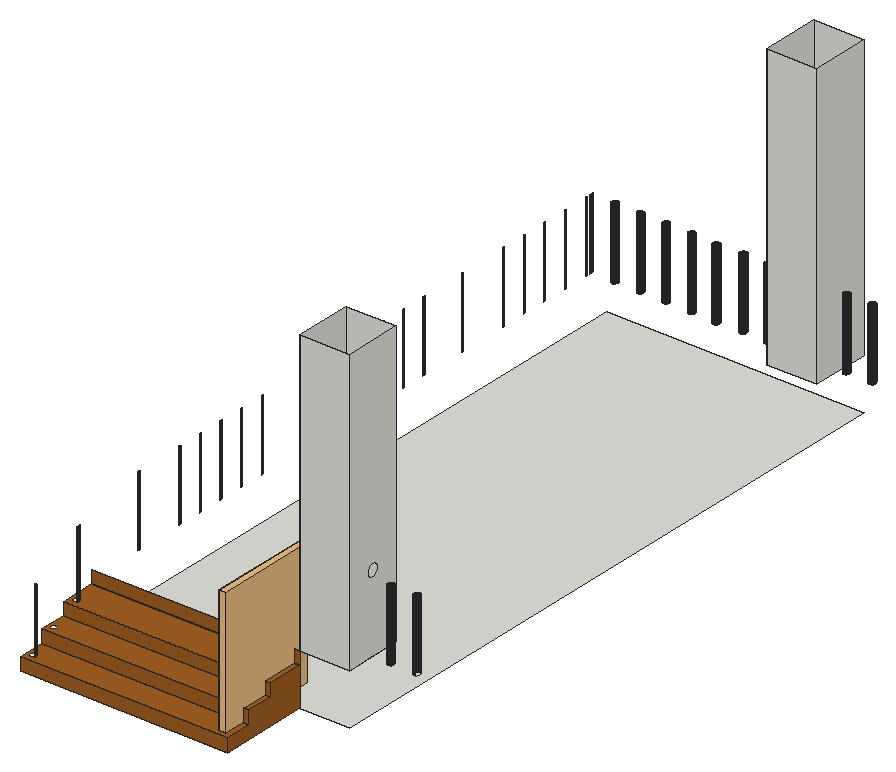
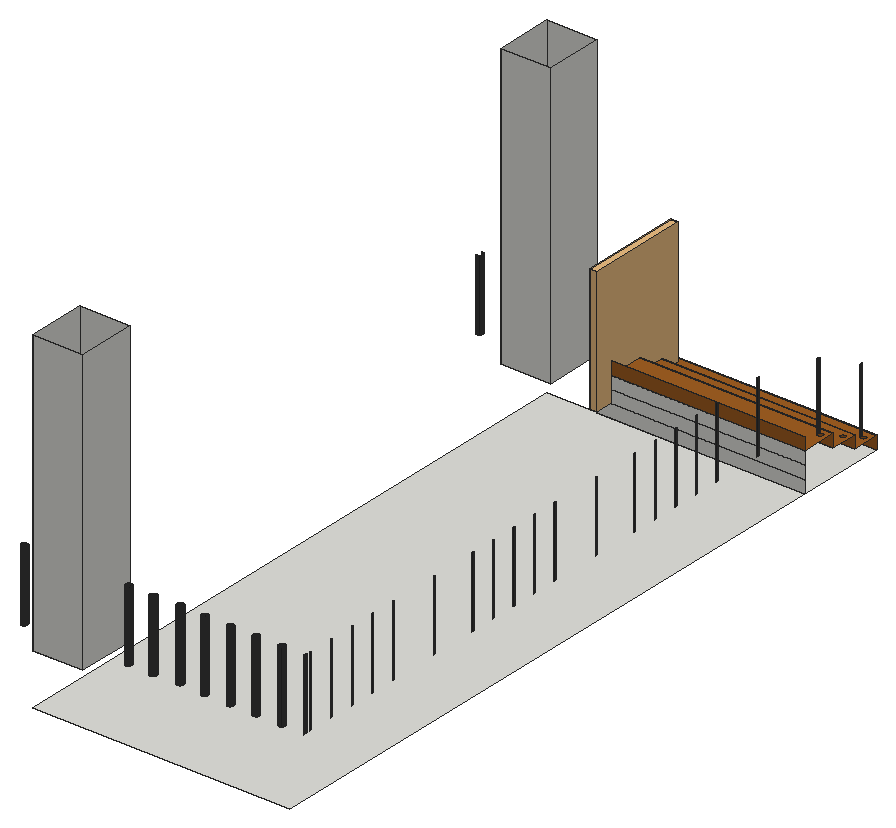
# SketchUp Ruby script. Lengths in inches.
U = 1.inch
M = Sketchup.active_model
def pt(a) = Geom::Point3d.new(a.map { |v| v * U })
def face(e, loops, mat)
  f = e.add_face(loops[0].map { |a| pt(a) })
  loops[1..].each { |l| e.add_face(l.map { |a| pt(a) }).erase! }
  f.material = f.back_material = mat if mat
  f
end
# faces: each face lists its corners as indices into pts; further lists are holes
def faces(e, pts, list, mat = nil) = list.each { |f| face(e, (f[0].is_a?(Array) ? f : [f]).map { |l| l.map { |i| pts[i] } }, mat) }
# xy, xz, yz: faces in a plane at the given z, y or x. An outline is a flat list of corners, or four numbers for a rectangle; further outlines are holes
def ring(l) = l.size == 4 ? [[l[0], l[1]], [l[2], l[1]], [l[2], l[3]], [l[0], l[3]]] : l.each_slice(2).to_a
def flat(e, list, mat, &to3) = list.each { |f| face(e, (f[0].is_a?(Array) ? f : [f]).map { |l| ring(l).map { |u, v| to3.(u, v) } }, mat) }
def xy(e, z, list, mat = nil) = flat(e, list, mat) { |x, y| [x, y, z] }
def xz(e, y, list, mat = nil) = flat(e, list, mat) { |x, z| [x, y, z] }
def yz(e, x, list, mat = nil) = flat(e, list, mat) { |y, z| [x, y, z] }
def lines(e, pts, list) = list.each { |a, b| e.add_line(pt(pts[a]), pt(pts[b])) }
# prism: a flat outline (further loops are holes) pulled along v
def prism(e, loops, v, mat = nil)
  f = face(e, loops, mat); d = Geom::Vector3d.new(v.map { |x| x * U })
  f.pushpull(f.normal.samedirection?(d) ? d.length : -d.length)
end
def box(e, o, s, mat = nil) = prism(e, [[o, [o[0] + s[0], o[1], o[2]], [o[0] + s[0], o[1] + s[1], o[2]], [o[0], o[1] + s[1], o[2]]]], [0, 0, s[2]], mat)
def at(x, y, z, deg = 0) = Geom::Transformation.translation(pt([x, y, z])) * Geom::Transformation.rotation(ORIGIN, Z_AXIS, deg.degrees)
def axes(o, x, y, z) = Geom::Transformation.new([*x, 0, *y, 0, *z, 0, *pt(o).to_a, 1])
def part(name) = M.definitions.add(name)
# library, detail: a bought-in or finely detailed component or shape, given as its bounding box
def library(name, o, s) = part(name).tap { |d| box(d.entities, o, s) }
def detail(e, o, s) = box(e.add_group.entities, o, s)
def put(e, d, t, mat = nil) = e.add_instance(d, t).tap { |i| i.material = mat if mat }
def group(e, t, mat = nil) = e.add_group.tap { |g| g.transformation = t; g.material = mat if mat }.entities
root = M.entities
M.materials.add("[0137_Black]").color = [45, 45, 45]
M.materials.add("[Wood Square Tile 02]").color = [160, 95, 34]
xy(root,0,[[0,0,193.3125,84],[0,84,240,684]])
xy(root,12,[[[0,0,193.3125,25.4375],[5.2,5.16,4.89,5.1875,4.58,5.25,4.28,5.34,3.99,5.47,3.72,5.62,3.46,5.8,3.23,6.01,3.01,6.24,2.83,6.49,2.67,6.76,2.53,7.05,2.43,7.35,2.37,7.65,2.33,7.96,2.33,8.28,2.36,8.59,2.42,8.9,2.51,9.2,2.64,9.49,2.79,9.76,2.97,10.02,3.18,10.25,3.41,10.47,3.66,10.65,3.93,10.8125,4.22,10.94,4.52,11.04,4.82,11.11,5.13,11.15,5.45,11.15,5.76,11.12,6.07,11.0625,6.37,10.97,6.66,10.84,6.93,10.6875,7.1875,10.51,7.42,10.3,7.63,10.07,7.82,9.82,7.98,9.55,8.11,9.26,8.21,8.96,8.28,8.66,8.32,8.34,8.32,8.03,8.29,7.72,8.23,7.41,8.14,7.11,8.01,6.82,7.86,6.55,7.68,6.29,7.47,6.06,7.24,5.84,6.99,5.66,6.71,5.5,6.43,5.37,6.13,5.27,5.83,5.2,5.51,5.16]]],"[Wood Square Tile 02]")
xy(root,24,[[[0,25.4375,193.3125,50.75],[4.7,30.03,4.39,30.06,4.08,30.12,3.78,30.22,3.49,30.34,3.22,30.49,2.96,30.68,2.73,30.88,2.51,31.11,2.33,31.37,2.17,31.64,2.04,31.92,1.9375,32.22,1.87,32.53,1.83,32.84,1.83,33.15,1.86,33.46,1.92,33.77,2.01,34.07,2.14,34.36,2.29,34.63,2.47,34.89,2.68,35.125,2.91,35.34,3.16,35.53,3.43,35.6875,3.72,35.82,4.02,35.92,4.32,35.99,4.63,36.02,4.95,36.03,5.26,36,5.57,35.93,5.87,35.84,6.16,35.72,6.43,35.5625,6.6875,35.38,6.92,35.17,7.14,34.94,7.32,34.6875,7.48,34.42,7.61,34.13,7.71,33.84,7.78,33.53,7.82,33.22,7.82,32.9,7.79,32.59,7.73,32.28,7.64,31.98,7.51,31.7,7.36,31.42,7.18,31.17,6.97,30.93,6.74,30.72,6.49,30.53,6.22,30.37,5.93,30.24,5.63,30.14,5.33,30.07,5.01,30.03]]],"[Wood Square Tile 02]")
xy(root,36,[[[0,50.75,193.3125,84],[5.56,55.09,5.25,55.12,4.94,55.18,4.64,55.27,4.35,55.4,4.08,55.55,3.82,55.74,3.59,55.94,3.375,56.17,3.1875,56.43,3.03,56.7,2.9,56.98,2.8,57.28,2.73,57.59,2.69,57.9,2.6875,58.21,2.72,58.52,2.78,58.83,2.87,59.13,3,59.42,3.15,59.69,3.33,59.95,3.54,60.19,3.77,60.4,4.02,60.59,4.29,60.75,4.58,60.875,4.875,60.98,5.18,61.05,5.49,61.08,5.81,61.08,6.12,61.06,6.43,60.99,6.73,60.9,7.02,60.78,7.29,60.62,7.55,60.4375,7.78,60.23,7.99,60,8.18,59.75,8.34,59.48,8.47,59.19,8.57,58.9,8.64,58.59,8.68,58.28,8.68,57.96,8.65,57.65,8.59,57.34,8.5,57.04,8.37,56.75,8.22,56.48,8.04,56.23,7.83,55.99,7.6,55.78,7.35,55.59,7.08,55.43,6.79,55.3,6.49,55.2,6.1875,55.13,5.875,55.09]]],"[Wood Square Tile 02]")
xy(root,48,[[193.3125,84,240,138.5625],[257.12,108.28,257.9,108.38,258.62,108.68,259.24,109.16,259.72,109.78,260.02,110.5,260.12,111.28,260.02,112.06,259.72,112.78,259.24,113.4,258.62,113.88,257.9,114.18,257.12,114.28,256.34,114.18,255.62,113.88,255,113.4,254.52,112.78,254.22,112.06,254.12,111.28,254.22,110.5,254.52,109.78,255,109.16,255.62,108.68,256.34,108.38],[281.12,108.28,280.34,108.38,279.62,108.68,279,109.16,278.52,109.78,278.22,110.5,278.12,111.28,278.22,112.06,278.52,112.78,279,113.4,279.62,113.88,280.34,114.18,281.12,114.28,281.9,114.18,282.62,113.88,283.24,113.4,283.72,112.78,284.02,112.06,284.12,111.28,284.02,110.5,283.72,109.78,283.24,109.16,282.62,108.68,281.9,108.38],[193.3125,629.4375,240,684],[246.01,653.72,246.79,653.82,247.51,654.12,248.13,654.6,248.61,655.22,248.91,655.94,249.01,656.72,243.01,656.72,243.11,655.94,243.41,655.22,243.89,654.6,244.51,654.12,245.23,653.82],
  [270.01,653.72,270.79,653.82,271.51,654.12,272.13,654.6,272.61,655.22,272.91,655.94,273.01,656.72,267.01,656.72,267.11,655.94,267.41,655.22,267.89,654.6,268.51,654.12,269.23,653.82],[243.01,656.72,249.01,656.72,248.91,657.5,248.61,658.22,248.13,658.84,247.51,659.32,246.79,659.62,246.01,659.72,245.23,659.62,244.51,659.32,243.89,658.84,243.41,658.22,243.11,657.5],[267.01,656.72,273.01,656.72,272.91,657.5,272.61,658.22,272.13,658.84,271.51,659.32,270.79,659.62,270.01,659.72,269.23,659.62,268.51,659.32,267.89,658.84,267.41,658.22,267.11,657.5]])
xz(root,0,[[0,0,193.3125,12]],"[Wood Square Tile 02]")
xz(root,25.4375,[[0,12,193.3125,24]],"[Wood Square Tile 02]")
xz(root,50.75,[[0,24,193.3125,36]],"[Wood Square Tile 02]")
xz(root,84,[[0,0,193.3125,12],[0,12,193.3125,24],[0,24,193.3125,36],[193.3125,48,240,312]])
xz(root,84,[[0,36,193.3125,48]],"[Wood Square Tile 02]")
xz(root,138.5625,[[193.3125,48,240,312]])
xz(root,629.4375,[[193.3125,48,240,312]])
xz(root,684,[[193.3125,48,240,312]])
yz(root,8.32,[[8.03,12,8.34,12,8.34,71.9,8.03,72.08]],"[0137_Black]")
yz(root,8.68,[[57.96,36,58.28,98.83]],"[0137_Black]")
yz(root,193.3125,[[84,48,138.5625,312],[629.4375,48,684,312]])
yz(root,193.3125,[[0,0,84,0,84,36,50.75,36,50.75,24,25.4375,24,25.4375,12,0,12]],"[Wood Square Tile 02]")
yz(root,240,[[84,48,111.28,48,111.28,114,110.65,114.03,110.03,114.13,109.43,114.29,108.84,114.52,108.28,114.8,107.75,115.15,107.27,115.54,106.82,115.99,106.43,116.47,106.09,117,105.8,117.56,105.57,118.15,105.41,118.75,105.3125,119.37,105.28,120,105.3125,120.63,105.41,121.25,105.57,121.85,105.8,122.44,106.09,123,106.43,123.53,106.82,124.01,107.27,124.46,107.75,124.85,108.28,125.2,108.84,125.48,109.43,125.71,110.03,125.87,110.65,125.97,111.28,126,111.91,125.97,112.53,125.87,113.14,125.71,113.72,125.48,114.28,125.2,114.81,124.85,115.3,124.46,115.74,124.01,116.14,123.53,116.48,123,116.76,122.44,116.99,121.85,117.15,121.25,117.25,120.63,117.28,120,117.25,119.37,117.15,118.75,116.99,118.15,116.76,117.56,116.48,117,116.14,116.47,115.74,115.99,115.3,115.54,114.81,115.15,114.28,114.8,113.72,114.52,113.14,114.29,112.53,114.13,111.91,114.03,111.28,114,111.28,48,138.5625,48,138.5625,312,84,312],[629.4375,48,684,312]])
p = [[8.01,6.82,12],[8.14,7.11,12],[8.14,7.11,72.59],[8.01,6.82,72.76],[8.23,7.41,12],[8.23,7.41,72.43],
  [8.29,7.72,12],[8.29,7.72,72.25],[8.32,8.03,12],[8.32,8.03,72.08],[8.32,8.34,12],[8.28,8.66,12],
  [8.28,8.66,71.72],[8.32,8.34,71.9],[8.21,8.96,12],[8.21,8.96,71.55],[8.11,9.26,12],[8.11,9.26,71.38],
  [7.98,9.55,12],[7.98,9.55,71.22],[8.04,56.23,36],[8.22,56.48,36],[8.22,56.48,98.83],[8.04,56.23,98.83],
  [8.37,56.75,36],[8.37,56.75,98.83],[8.5,57.04,36],[8.5,57.04,98.83],[8.59,57.34,36],[8.59,57.34,98.83],
  [8.65,57.65,36],[8.65,57.65,98.83],[8.68,57.96,36],[8.68,57.96,98.83],[8.68,58.28,36],[8.64,58.59,36],
  [8.64,58.59,98.83],[8.68,58.28,98.83],[8.57,58.9,36],[8.57,58.9,98.83],[8.47,59.19,36],[8.47,59.19,98.83],
  [8.34,59.48,36],[8.34,59.48,98.83],[8.18,59.75,36],[8.18,59.75,98.83],[7.99,60,36],[7.99,60,98.83],
  [256.34,108.38,48],[257.12,108.28,48],[257.12,108.28,113.8],[256.34,108.38,113.8],[257.9,108.38,48],[257.9,108.38,113.8],
  [280.34,108.38,48],[281.12,108.28,48],[281.12,108.28,113.8],[280.34,108.38,113.8],[281.9,108.38,48],[281.9,108.38,113.8],
  [255.62,108.68,48],[255.62,108.68,113.8],[258.62,108.68,48],[258.62,108.68,113.8],[279.62,108.68,48],[279.62,108.68,113.8],
  [255,109.16,48],[255,109.16,113.8],[259.24,109.16,48],[259.24,109.16,113.8],[279,109.16,48],[279,109.16,113.8],
  [254.52,109.78,48],[254.52,109.78,113.8],[259.72,109.78,48],[259.72,109.78,113.8],[278.52,109.78,48],[278.52,109.78,113.8],
  [254.22,110.5,48],[254.22,110.5,113.8],[260.02,110.5,48],[260.02,110.5,113.8],[278.22,110.5,48],[278.22,110.5,113.8],
  [254.12,111.28,48],[254.12,111.28,113.8],[260.12,111.28,48],[260.12,111.28,113.8],[278.12,111.28,48],[278.12,111.28,113.8],
  [254.22,112.06,48],[254.22,112.06,113.8],[260.02,112.06,48],[260.02,112.06,113.8],[278.22,112.06,48],[278.22,112.06,113.8],
  [254.52,112.78,48],[254.52,112.78,113.8],[259.72,112.78,48],[259.72,112.78,113.8],[278.52,112.78,48],[278.52,112.78,113.8],
  [255,113.4,48],[255,113.4,113.8],[259.24,113.4,48],[259.24,113.4,113.8],[279,113.4,48],[279,113.4,113.8],
  [255.62,113.88,48],[255.62,113.88,113.8],[258.62,113.88,48],[258.62,113.88,113.8],[279.62,113.88,48],[279.62,113.88,113.8],
  [256.34,114.18,48],[256.34,114.18,113.8],[257.9,114.18,48],[257.9,114.18,113.8],[280.34,114.18,48],[280.34,114.18,113.8],
  [282.62,113.88,48],[281.9,114.18,48],[281.9,114.18,113.8],[282.62,113.88,113.8],[257.12,114.28,48],[257.12,114.28,113.8],
  [281.12,114.28,48],[281.12,114.28,113.8],[7.9,127.49,48],[8,128.27,48],[8,128.27,113.8],[7.9,127.49,113.8],
  [7.9,129.05,48],[7.9,129.05,113.8],[7.9,175.49,48],[8,176.27,48],[8,176.27,113.8],[7.9,175.49,113.8],
  [7.9,177.05,48],[7.9,177.05,113.8],[7.9,199.49,48],[8,200.27,48],[8,200.27,113.8],[7.9,199.49,113.8],
  [7.9,201.05,48],[7.9,201.05,113.8],[7.9,223.49,48],[8,224.27,48],[8,224.27,113.8],[7.9,223.49,113.8],
  [7.9,225.05,48],[7.9,225.05,113.8],[7.9,247.49,48],[8,248.27,48],[8,248.27,113.8],[7.9,247.49,113.8],
  [7.9,249.05,48],[7.9,249.05,113.8],[7.9,271.49,48],[8,272.27,48],[8,272.27,113.8],[7.9,271.49,113.8],
  [7.9,273.05,48],[7.9,273.05,113.8],[7.9,316.38,48],[8,317.16,48],[8,317.16,113.8],[7.9,316.38,113.8],
  [7.9,317.93,48],[7.9,317.93,113.8],[7.9,364.38,48],[8,365.16,48],[8,365.16,113.8],[7.9,364.38,113.8],
  [7.9,365.93,48],[7.9,365.93,113.8],[7.9,388.38,48],[8,389.16,48],[8,389.16,113.8],[7.9,388.38,113.8],
  [7.9,389.93,48],[7.9,389.93,113.8],[7.9,412.38,48],[8,413.16,48],[8,413.16,113.8],[7.9,412.38,113.8],
  [7.9,413.93,48],[7.9,413.93,113.8],[7.9,436.38,48],[8,437.16,48],[8,437.16,113.8],[7.9,436.38,113.8],
  [7.9,437.93,48],[7.9,437.93,113.8],[7.9,460.38,48],[8,461.16,48],[8,461.16,113.8],[7.9,460.38,113.8],
  [7.9,461.93,48],[7.9,461.93,113.8],[7.9,505.27,48],[8,506.05,48],[8,506.05,113.8],[7.9,505.27,113.8],
  [7.9,506.82,48],[7.9,506.82,113.8],[7.9,553.27,48],[8,554.05,48],[8,554.05,113.8],[7.9,553.27,113.8],
  [7.9,554.82,48],[7.9,554.82,113.8],[7.9,577.27,48],[8,578.05,48],[8,578.05,113.8],[7.9,577.27,113.8],
  [7.9,578.82,48],[7.9,578.82,113.8],[7.9,601.27,48],[8,602.05,48],[8,602.05,113.8],[7.9,601.27,113.8],
  [7.9,602.82,48],[7.9,602.82,113.8],[7.9,625.27,48],[8,626.05,48],[8,626.05,113.8],[7.9,625.27,113.8],
  [7.9,626.82,48],[7.9,626.82,113.8],[8,650.05,48],[7.9,650.82,48],[7.9,650.82,113.8],[8,650.05,113.8],
  [124.86,652.27,48],[125.63,652.17,48],[125.63,652.17,113.8],[124.86,652.27,113.8],[126.41,652.27,48],[126.41,652.27,113.8],
  [124.13,652.57,48],[124.13,652.57,113.8],[127.13,652.57,48],[127.13,652.57,113.8],[123.51,653.04,48],[123.51,653.04,113.8],
  [127.76,653.04,48],[127.76,653.04,113.8],[123.04,653.67,48],[123.04,653.67,113.8],[128.23,653.67,48],[128.23,653.67,113.8],
  [172.38,653.2,48],[173.16,653.1,48],[173.16,653.1,113.8],[172.38,653.2,113.8],[173.93,653.2,48],[173.93,653.2,113.8],
  [171.66,653.5,48],[171.66,653.5,113.8],[174.66,653.5,48],[174.66,653.5,113.8],[171.04,653.98,48],[171.04,653.98,113.8],
  [175.28,653.98,48],[175.28,653.98,113.8],[28.86,653.82,48],[29.63,653.72,48],[29.63,653.72,113.8],[28.86,653.82,113.8],
  [30.41,653.82,48],[30.41,653.82,113.8],[52.86,653.82,48],[53.63,653.72,48],[53.63,653.72,113.8],[52.86,653.82,113.8],
  [54.41,653.82,48],[54.41,653.82,113.8],[76.86,653.82,48],[77.63,653.72,48],[77.63,653.72,113.8],[76.86,653.82,113.8],
  [78.41,653.82,48],[78.41,653.82,113.8],[100.86,653.82,48],[101.63,653.72,48],[101.63,653.72,113.8],[100.86,653.82,113.8],
  [102.41,653.82,48],[102.41,653.82,113.8],[122.74,654.39,48],[122.74,654.39,113.8],[128.53,654.39,48],[128.53,654.39,113.8],
  [148.86,653.82,48],[149.63,653.72,48],[149.63,653.72,113.8],[148.86,653.82,113.8],[150.41,653.82,48],[150.41,653.82,113.8],
  [245.23,653.82,48],[246.01,653.72,48],[246.01,653.72,113.8],[245.23,653.82,113.8],[246.79,653.82,48],[246.79,653.82,113.8],
  [269.23,653.82,48],[270.01,653.72,48],[270.01,653.72,113.8],[269.23,653.82,113.8],[270.79,653.82,48],[270.79,653.82,113.8],
  [28.13,654.12,48],[28.13,654.12,113.8],[31.13,654.12,48],[31.13,654.12,113.8],[52.13,654.12,48],[52.13,654.12,113.8],
  [55.13,654.12,48],[55.13,654.12,113.8],[76.13,654.12,48],[76.13,654.12,113.8],[79.13,654.12,48],[79.13,654.12,113.8],
  [100.13,654.12,48],[100.13,654.12,113.8],[103.13,654.12,48],[103.13,654.12,113.8],[148.13,654.12,48],[148.13,654.12,113.8],
  [151.13,654.12,48],[151.13,654.12,113.8],[244.51,654.12,48],[244.51,654.12,113.8],[247.51,654.12,48],[247.51,654.12,113.8],
  [268.51,654.12,48],[268.51,654.12,113.8],[271.51,654.12,48],[271.51,654.12,113.8],[170.56,654.6,48],[170.56,654.6,113.8],
  [175.76,654.6,48],[175.76,654.6,113.8],[27.51,654.6,48],[27.51,654.6,113.8],[31.76,654.6,48],[31.76,654.6,113.8],
  [51.51,654.6,48],[51.51,654.6,113.8],[55.76,654.6,48],[55.76,654.6,113.8],[75.51,654.6,48],[75.51,654.6,113.8],
  [79.76,654.6,48],[79.76,654.6,113.8],[99.51,654.6,48],[99.51,654.6,113.8],[103.76,654.6,48],[103.76,654.6,113.8],
  [147.51,654.6,48],[147.51,654.6,113.8],[151.76,654.6,48],[151.76,654.6,113.8],[243.89,654.6,48],[243.89,654.6,113.8],
  [248.13,654.6,48],[248.13,654.6,113.8],[267.89,654.6,48],[267.89,654.6,113.8],[272.13,654.6,48],[272.13,654.6,113.8],
  [122.63,655.17,48],[122.63,655.17,113.8],[122.63,655.17,113.71],[128.63,655.17,48],[128.63,655.17,113.71],[128.63,655.17,113.8],
  [7.76,654.6,48],[8.23,655.22,48],[8.23,655.22,113.8],[7.76,654.6,113.8],[27.04,655.22,48],[27.04,655.22,113.8],
  [32.23,655.22,48],[32.23,655.22,113.8],[51.04,655.22,48],[51.04,655.22,113.8],[56.23,655.22,48],[56.23,655.22,113.8],
  [75.04,655.22,48],[75.04,655.22,113.8],[80.23,655.22,48],[80.23,655.22,113.8],[99.04,655.22,48],[99.04,655.22,113.8],
  [104.23,655.22,48],[104.23,655.22,113.8],[147.04,655.22,48],[147.04,655.22,113.8],[152.23,655.22,48],[152.23,655.22,113.8],
  [170.26,655.32,48],[170.26,655.32,113.8],[176.05,655.32,48],[176.05,655.32,113.8],[243.41,655.22,48],[243.41,655.22,113.8],
  [248.61,655.22,48],[248.61,655.22,113.8],[267.41,655.22,48],[267.41,655.22,113.8],[272.61,655.22,48],[272.61,655.22,113.8],
  [8.53,655.94,48],[8.53,655.94,113.61],[8.53,655.94,113.8],[26.74,655.94,48],[26.74,655.94,113.8],[26.74,655.94,113.61],
  [32.53,655.94,48],[32.53,655.94,113.61],[32.53,655.94,113.8],[50.74,655.94,48],[50.74,655.94,113.8],[50.74,655.94,113.61],
  [56.53,655.94,48],[56.53,655.94,113.61],[56.53,655.94,113.8],[74.74,655.94,48],[74.74,655.94,113.8],[74.74,655.94,113.61],
  [80.53,655.94,48],[80.53,655.94,113.61],[80.53,655.94,113.8],[98.74,655.94,48],[98.74,655.94,113.8],[98.74,655.94,113.61],
  [104.53,655.94,48],[104.53,655.94,113.61],[104.53,655.94,113.8],[122.74,655.94,48],[122.74,655.94,113.8],[122.74,655.94,113.61],
  [128.53,655.94,48],[128.53,655.94,113.61],[128.53,655.94,113.8],[146.74,655.94,48],[146.74,655.94,113.8],[146.74,655.94,113.61],
  [152.53,655.94,48],[152.53,655.94,113.61],[152.53,655.94,113.8],[243.11,655.94,48],[243.11,655.94,113.8],[243.11,655.94,113.61],
  [248.91,655.94,48],[248.91,655.94,113.61],[248.91,655.94,113.8],[267.11,655.94,48],[267.11,655.94,113.8],[267.11,655.94,113.61],
  [272.91,655.94,48],[272.91,655.94,113.61],[272.91,655.94,113.8],[170.16,656.1,48],[170.16,656.1,113.8],[176.16,656.1,48],
  [176.16,656.1,113.8],[8.63,656.72,48],[8.63,656.72,113.71],[8.63,656.72,113.8],[26.63,656.72,48],[26.63,656.72,113.8],
  [26.63,656.72,113.71],[32.63,656.72,48],[32.63,656.72,113.71],[32.63,656.72,113.8],[50.63,656.72,48],[50.63,656.72,113.8],
  [50.63,656.72,113.71],[56.63,656.72,48],[56.63,656.72,113.71],[56.63,656.72,113.8],[74.63,656.72,48],[74.63,656.72,113.8],
  [74.63,656.72,113.71],[80.63,656.72,48],[80.63,656.72,113.71],[80.63,656.72,113.8],[98.63,656.72,48],[98.63,656.72,113.8],
  [98.63,656.72,113.71],[104.63,656.72,48],[104.63,656.72,113.71],[104.63,656.72,113.8],[123.04,656.67,48],[123.04,656.67,113.8],
  [128.23,656.67,48],[128.23,656.67,113.8],[146.63,656.72,48],[146.63,656.72,113.8],[146.63,656.72,113.71],[152.63,656.72,48],
  [152.63,656.72,113.71],[152.63,656.72,113.8],[243.01,656.72,48],[243.01,656.72,113.8],[249.01,656.72,48],[249.01,656.72,113.71],
  [249.01,656.72,113.8],[267.01,656.72,48],[267.01,656.72,113.8],[267.01,656.72,113.71],[273.01,656.72,48],[273.01,656.72,113.71],
  [273.01,656.72,113.8],[170.26,656.875,48],[170.24,656.72,48],[170.26,656.875,113.8],[176.08,656.72,48],[176.05,656.875,48],
  [176.05,656.875,113.8],[8.53,657.5,48],[8.53,657.5,113.8],[26.74,657.5,48],[26.74,657.5,113.8],[32.53,657.5,48],
  [32.53,657.5,113.8],[50.74,657.5,48],[50.74,657.5,113.8],[56.53,657.5,48],[56.53,657.5,113.8],[74.74,657.5,48],
  [74.74,657.5,113.8],[80.53,657.5,48],[80.53,657.5,113.8],[98.74,657.5,48],[98.74,657.5,113.8],[104.53,657.5,48],
  [104.53,657.5,113.8],[123.51,657.29,48],[123.08,656.72,48],[123.51,657.29,113.8],[128.19,656.72,48],[127.76,657.29,48],
  [127.76,657.29,113.8],[146.74,657.5,48],[146.74,657.5,113.8],[152.53,657.5,48],[152.53,657.5,113.8],[243.11,657.5,48],
  [243.11,657.5,113.8],[248.91,657.5,48],[248.91,657.5,113.8],[267.11,657.5,48],[267.11,657.5,113.8],[272.91,657.5,48],
  [272.91,657.5,113.8],[170.56,657.6,48],[170.56,657.6,113.8],[175.76,657.6,48],[175.76,657.6,113.8],[124.13,657.76,48],
  [124.13,657.76,113.8],[127.13,657.76,48],[127.13,657.76,113.8],[8.23,658.22,48],[8.23,658.22,113.8],[27.04,658.22,48],
  [27.04,658.22,113.8],[32.23,658.22,48],[32.23,658.22,113.8],[51.04,658.22,48],[51.04,658.22,113.8],[56.23,658.22,48],
  [56.23,658.22,113.8],[75.04,658.22,48],[75.04,658.22,113.8],[80.23,658.22,48],[80.23,658.22,113.8],[99.04,658.22,48],
  [99.04,658.22,113.8],[104.23,658.22,48],[104.23,658.22,113.8],[147.04,658.22,48],[147.04,658.22,113.8],[152.23,658.22,48],
  [152.23,658.22,113.8],[243.41,658.22,48],[243.41,658.22,113.8],[248.61,658.22,48],[248.61,658.22,113.8],[267.41,658.22,48],
  [267.41,658.22,113.8],[272.61,658.22,48],[272.61,658.22,113.8],[171.04,658.22,48],[171.04,658.22,113.8],[175.28,658.22,48],
  [175.28,658.22,113.8],[124.86,658.0625,48],[124.86,658.0625,113.8],[126.41,658.0625,48],[126.41,658.0625,113.8],[125.63,658.17,48],
  [125.63,658.17,113.8],[7.76,658.84,48],[7.76,658.84,113.8],[27.51,658.84,48],[27.51,658.84,113.8],[31.76,658.84,48],
  [31.76,658.84,113.8],[51.51,658.84,48],[51.51,658.84,113.8],[55.76,658.84,48],[55.76,658.84,113.8],[75.51,658.84,48],
  [75.51,658.84,113.8],[79.76,658.84,48],[79.76,658.84,113.8],[99.51,658.84,48],[99.51,658.84,113.8],[103.76,658.84,48],
  [103.76,658.84,113.8],[147.51,658.84,48],[147.51,658.84,113.8],[151.76,658.84,48],[151.76,658.84,113.8],[171.66,658.7,48],
  [171.66,658.7,113.8],[174.66,658.7,48],[174.66,658.7,113.8],[243.89,658.84,48],[243.89,658.84,113.8],[248.13,658.84,48],
  [248.13,658.84,113.8],[267.89,658.84,48],[267.89,658.84,113.8],[272.13,658.84,48],[272.13,658.84,113.8],[172.38,659,48],
  [172.38,659,113.8],[173.93,659,48],[173.93,659,113.8],[28.13,659.32,48],[28.13,659.32,113.8],[31.13,659.32,48],
  [31.13,659.32,113.8],[52.13,659.32,48],[52.13,659.32,113.8],[55.13,659.32,48],[55.13,659.32,113.8],[76.13,659.32,48],
  [76.13,659.32,113.8],[79.13,659.32,48],[79.13,659.32,113.8],[100.13,659.32,48],[100.13,659.32,113.8],[103.13,659.32,48],
  [103.13,659.32,113.8],[148.13,659.32,48],[148.13,659.32,113.8],[151.13,659.32,48],[151.13,659.32,113.8],[244.51,659.32,48],
  [244.51,659.32,113.8],[247.51,659.32,48],[247.51,659.32,113.8],[268.51,659.32,48],[268.51,659.32,113.8],[271.51,659.32,48],
  [271.51,659.32,113.8],[173.16,659.1,48],[173.16,659.1,113.8],[28.86,659.62,48],[28.86,659.62,113.8],[30.41,659.62,48],
  [30.41,659.62,113.8],[52.86,659.62,48],[52.86,659.62,113.8],[54.41,659.62,48],[54.41,659.62,113.8],[76.86,659.62,48],
  [76.86,659.62,113.8],[78.41,659.62,48],[78.41,659.62,113.8],[100.86,659.62,48],[100.86,659.62,113.8],[102.41,659.62,48],
  [102.41,659.62,113.8],[148.86,659.62,48],[148.86,659.62,113.8],[150.41,659.62,48],[150.41,659.62,113.8],[245.23,659.62,48],
  [245.23,659.62,113.8],[246.79,659.62,48],[246.79,659.62,113.8],[269.23,659.62,48],[269.23,659.62,113.8],[270.79,659.62,48],
  [270.79,659.62,113.8],[29.63,659.72,48],[29.63,659.72,113.8],[53.63,659.72,48],[53.63,659.72,113.8],[77.63,659.72,48],
  [77.63,659.72,113.8],[101.63,659.72,48],[101.63,659.72,113.8],[149.63,659.72,48],[149.63,659.72,113.8],[246.01,659.72,48],
  [246.01,659.72,113.8],[270.01,659.72,48],[270.01,659.72,113.8],[281.12,111.28,48],[281.12,111.28,113.8],[257.12,111.28,48],
  [257.12,111.28,113.58]]
faces(root,p,[[0,1,2,3],[1,4,5,2],[4,6,7,5],[6,8,9,7],[10,11,12,13],[11,14,15,12],[14,16,17,15],[16,18,19,17],
  [20,21,22,23],[21,24,25,22],[24,26,27,25],[26,28,29,27],[28,30,31,29],[30,32,33,31],[34,35,36,37],[35,38,39,36],
  [38,40,41,39],[40,42,43,41],[42,44,45,43],[44,46,47,45],[48,49,50,51],[49,52,53,50],[54,55,56,57],[55,58,59,56],
  [60,48,51,61],[52,62,63,53],[64,54,57,65],[66,60,61,67],[62,68,69,63],[70,64,65,71],[72,66,67,73],[68,74,75,69],
  [76,70,71,77],[78,72,73,79],[74,80,81,75],[82,76,77,83],[84,78,79,85],[80,86,87,81],[88,82,83,89],[90,84,85,91],
  [86,92,93,87],[94,88,89,95],[96,90,91,97],[92,98,99,93],[100,94,95,101],[102,96,97,103],[98,104,105,99],[106,100,101,107],
  [108,102,103,109],[104,110,111,105],[112,106,107,113],[114,108,109,115],[110,116,117,111],[118,112,113,119],[120,121,122,123],[124,114,115,125],
  [116,124,125,117],[126,118,119,127],[121,126,127,122],[128,129,130,131],[129,132,133,130],[134,135,136,137],[135,138,139,136],[140,141,142,143],
  [141,144,145,142],[146,147,148,149],[147,150,151,148],[152,153,154,155],[153,156,157,154],[158,159,160,161],[159,162,163,160],[164,165,166,167],
  [165,168,169,166],[170,171,172,173],[171,174,175,172],[176,177,178,179],[177,180,181,178],[182,183,184,185],[183,186,187,184],[188,189,190,191],
  [189,192,193,190],[194,195,196,197],[195,198,199,196],[200,201,202,203],[201,204,205,202],[206,207,208,209],[207,210,211,208],[212,213,214,215],
  [213,216,217,214],[218,219,220,221],[219,222,223,220],[224,225,226,227],[225,228,229,226],[230,231,232,233],[234,235,236,237],[235,238,239,236],
  [240,234,237,241],[238,242,243,239],[244,240,241,245],[242,246,247,243],[248,244,245,249],[246,250,251,247],[252,253,254,255],[253,256,257,254],
  [258,252,255,259],[256,260,261,257],[262,258,259,263],[260,264,265,261],[266,267,268,269],[267,270,271,268],[272,273,274,275],[273,276,277,274],
  [278,279,280,281],[279,282,283,280],[284,285,286,287],[285,288,289,286],[290,248,249,291],[250,292,293,251],[294,295,296,297],[295,298,299,296],
  [300,301,302,303],[301,304,305,302],[306,307,308,309],[307,310,311,308],[312,266,269,313],[270,314,315,271],[316,272,275,317],[276,318,319,277],
  [320,278,281,321],[282,322,323,283],[324,284,287,325],[288,326,327,289],[328,294,297,329],[298,330,331,299],[332,300,303,333],[304,334,335,305],
  [336,306,309,337],[310,338,339,311],[340,262,263,341],[264,342,343,265],[344,312,313,345],[314,346,347,315],[348,316,317,349],[318,350,351,319],
  [352,320,321,353],[322,354,355,323],[356,324,325,357],[326,358,359,327],[360,328,329,361],[330,362,363,331],[364,332,333,365],[334,366,367,335],
  [368,336,337,369],[338,370,371,339],[372,290,291,373,374],[292,375,376,377,293],[378,379,380,381],[382,344,345,383],[346,384,385,347],[386,348,349,387],
  [350,388,389,351],[390,352,353,391],[354,392,393,355],[394,356,357,395],[358,396,397,359],[398,360,361,399],[362,400,401,363],[402,340,341,403],
  [342,404,405,343],[406,364,365,407],[366,408,409,367],[410,368,369,411],[370,412,413,371],[379,414,415,416,380],[417,382,383,418,419],[384,420,421,422,385],
  [423,386,387,424,425],[388,426,427,428,389],[429,390,391,430,431],[392,432,433,434,393],[435,394,395,436,437],[396,438,439,440,397],[441,372,374,373,442,443],[375,444,445,446,377,376],
  [447,398,399,448,449],[400,450,451,452,401],[453,406,407,454,455],[408,456,457,458,409],[459,410,411,460,461],[412,462,463,464,413],[465,402,403,466],[404,467,468,405],
  [414,469,470,471,416,415],[472,417,419,418,473,474],[420,475,476,477,422,421],[478,423,425,424,479,480],[426,481,482,483,428,427],[484,429,431,430,485,486],[432,487,488,489,434,433],[490,435,437,436,491,492],
  [438,493,494,495,440,439],[496,441,443,442,497],[444,498,499,446,445],[500,447,449,448,501,502],[450,503,504,505,452,451],[506,453,455,454,507],[456,508,509,510,458,457],[511,459,461,460,512,513],
  [462,514,515,516,464,463],[517,518,465,466,519],[467,520,521,522,468],[469,523,524,471,470],[525,472,474,473,526],[475,527,528,477,476],[529,478,480,479,530],[481,531,532,483,482],
  [533,484,486,485,534],[487,535,536,489,488],[537,490,492,491,538],[493,539,540,495,494],[541,542,496,497,543],[498,544,545,546,499],[547,500,502,501,548],[503,549,550,505,504],
  [551,506,507,552],[508,553,554,510,509],[555,511,513,512,556],[514,557,558,516,515],[559,517,519,560],[521,561,562,522],[563,541,543,564],[545,565,566,546],
  [523,567,568,524],[569,525,526,570],[527,571,572,528],[573,529,530,574],[531,575,576,532],[577,533,534,578],[535,579,580,536],[581,537,538,582],
  [539,583,584,540],[585,547,548,586],[549,587,588,550],[589,551,552,590],[553,591,592,554],[593,555,556,594],[557,595,596,558],[597,559,560,598],
  [561,599,600,562],[601,563,564,602],[565,603,604,566],[605,601,602,606],[603,605,606,604],[567,607,608,568],[609,569,570,610],[571,611,612,572],
  [613,573,574,614],[575,615,616,576],[617,577,578,618],[579,619,620,580],[621,581,582,622],[583,623,624,584],[625,585,586,626],[587,627,628,588],
  [629,597,598,630],[599,631,632,600],[633,589,590,634],[591,635,636,592],[637,593,594,638],[595,639,640,596],[641,629,630,642],[631,643,644,632],
  [645,609,610,646],[611,647,648,612],[649,613,614,650],[615,651,652,616],[653,617,618,654],[619,655,656,620],[657,621,622,658],[623,659,660,624],
  [661,625,626,662],[627,663,664,628],[665,633,634,666],[635,667,668,636],[669,637,638,670],[639,671,672,640],[673,641,642,674],[643,673,674,644],
  [675,645,646,676],[647,677,678,648],[679,649,650,680],[651,681,682,652],[683,653,654,684],[655,685,686,656],[687,657,658,688],[659,689,690,660],
  [691,661,662,692],[663,693,694,664],[695,665,666,696],[667,697,698,668],[699,669,670,700],[671,701,702,672],[703,675,676,704],[677,703,704,678],
  [705,679,680,706],[681,705,706,682],[707,683,684,708],[685,707,708,686],[709,687,688,710],[689,709,710,690],[711,691,692,712],[693,711,712,694],
  [713,695,696,714],[697,713,714,698],[715,699,700,716],[701,715,716,702]],"[0137_Black]")
lines(root,p,[[717,718],[719,720]])
detail(root,[180.89,30.03,24],[5.99,6,58.48])
detail(root,[180.82,5.16,12],[6.92,94.91,117.02])
